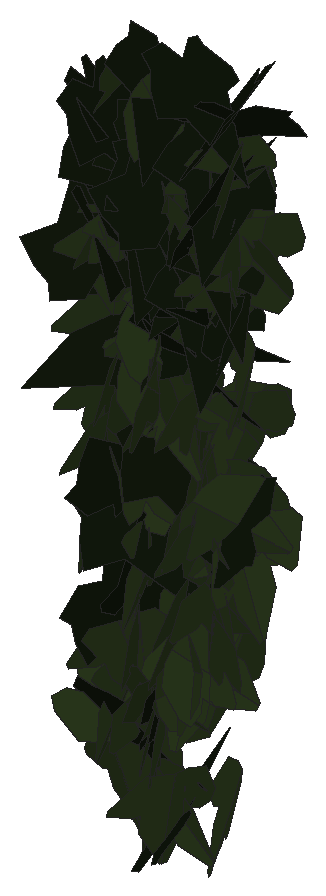
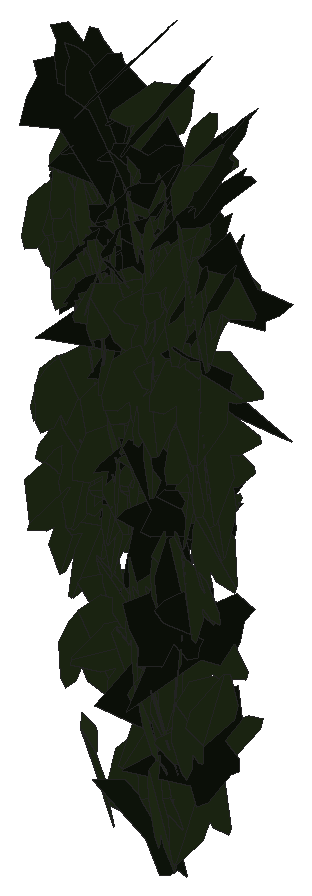
# SketchUp Ruby script. Lengths in inches.
U = 1.inch
M = Sketchup.active_model
def pt(a) = Geom::Point3d.new(a.map { |v| v * U })
def face(e, loops, mat)
  f = e.add_face(loops[0].map { |a| pt(a) })
  loops[1..].each { |l| e.add_face(l.map { |a| pt(a) }).erase! }
  f.material = f.back_material = mat if mat
  f
end
# faces: each face lists its corners as indices into pts; further lists are holes
def faces(e, pts, list, mat = nil) = list.each { |f| face(e, (f[0].is_a?(Array) ? f : [f]).map { |l| l.map { |i| pts[i] } }, mat) }
# xy, xz, yz: faces in a plane at the given z, y or x. An outline is a flat list of corners, or four numbers for a rectangle; further outlines are holes
def ring(l) = l.size == 4 ? [[l[0], l[1]], [l[2], l[1]], [l[2], l[3]], [l[0], l[3]]] : l.each_slice(2).to_a
def flat(e, list, mat, &to3) = list.each { |f| face(e, (f[0].is_a?(Array) ? f : [f]).map { |l| ring(l).map { |u, v| to3.(u, v) } }, mat) }
def xy(e, z, list, mat = nil) = flat(e, list, mat) { |x, y| [x, y, z] }
def xz(e, y, list, mat = nil) = flat(e, list, mat) { |x, z| [x, y, z] }
def yz(e, x, list, mat = nil) = flat(e, list, mat) { |y, z| [x, y, z] }
def lines(e, pts, list) = list.each { |a, b| e.add_line(pt(pts[a]), pt(pts[b])) }
# prism: a flat outline (further loops are holes) pulled along v
def prism(e, loops, v, mat = nil)
  f = face(e, loops, mat); d = Geom::Vector3d.new(v.map { |x| x * U })
  f.pushpull(f.normal.samedirection?(d) ? d.length : -d.length)
end
def box(e, o, s, mat = nil) = prism(e, [[o, [o[0] + s[0], o[1], o[2]], [o[0] + s[0], o[1] + s[1], o[2]], [o[0], o[1] + s[1], o[2]]]], [0, 0, s[2]], mat)
def at(x, y, z, deg = 0) = Geom::Transformation.translation(pt([x, y, z])) * Geom::Transformation.rotation(ORIGIN, Z_AXIS, deg.degrees)
def axes(o, x, y, z) = Geom::Transformation.new([*x, 0, *y, 0, *z, 0, *pt(o).to_a, 1])
def part(name) = M.definitions.add(name)
# library, detail: a bought-in or finely detailed component or shape, given as its bounding box
def library(name, o, s) = part(name).tap { |d| box(d.entities, o, s) }
def detail(e, o, s) = box(e.add_group.entities, o, s)
def put(e, d, t, mat = nil) = e.add_instance(d, t).tap { |i| i.material = mat if mat }
def group(e, t, mat = nil) = e.add_group.tap { |g| g.transformation = t; g.material = mat if mat }.entities
root = M.entities
M.materials.add("efeu1").color = [18, 25, 13]
M.materials.add("efeu2").color = [43, 57, 29]
c1 = part("ivyleaf_10")
p = [[0,0.5,-0.03],[-0.0625,2.02,-0.43],[-0.19,2.01,-0.46],[-0.54,1.05,-0.29],[-0.52,0.625,-0.18],[-0.83,0.76,-0.28],
  [-1.16,0.64,-0.33],[-1.15,0.33,-0.24],[-0.77,-0.39,0.02],[-0.3,-0.51,0.16],[0.04,-0.48,0.23],[-0.02,2.01,-0.4375],
  [-0.06,2.01,-0.43],[0.04,-0.49,0.23],[0.67,-0.49,0.14],[1.38,0.36,-0.2],[1.375,0.51,-0.24],[0.81,0.65,-0.19],
  [0.62,0.59,-0.15],[0.6,1.09,-0.28],[0.5,1.23,-0.31]]
faces(c1.entities,p,[[0,1,2,3,4,5,6,7,8,9,10],[11,12,0,13,14,15,16,17,18,19,20]],"efeu2")
c2 = part("ivyleaf_9")
p = [[1.54,2.16,1.25],[1.36,2.04,1.19],[-0.21,0.99,0.68],[-0.71,1.11,0.82],[-0.85,0.86,0.67],[-0.8,0.17,0.21],
  [-0.9,-0.01,0.1],[-0.67,-0.16,-0.02],[-0.08,-0.08,-0.05],[-0.03,-0.6,-0.4],[0.65,-0.88,-0.66],[0.83,-0.6,-0.49],
  [1.29,-0.42,-0.43],[1.8125,-0.07,-0.26],[1.21,0.44,0.15]]
faces(c2.entities,p,[[0,1,2,3,4,5,6,7,8,9,10,11,12,13,14]],"efeu1")
put(root,c1,axes([25.26,224.34,221.76],[0.24125,-0.40077,-0.17658],[-0.09619,0.14819,-0.46775],[0.42726,0.25966,-0.0056]))
put(root,c2,axes([24.83,224.32,221.36],[-0.37536,-0.25401,0.21115],[0.19137,0.09328,0.45241],[-0.26923,0.42045,0.02719]))
put(root,c1,axes([25.51,224.54,222.11],[0.27688,-0.39865,0.12008],[0.06912,-0.0982,-0.48537],[0.41056,0.28537,0.00073]))
put(root,c1,axes([24.86,224.34,221.39],[-0.44159,0.20009,0.12234],[-0.14457,-0.02688,-0.47789],[-0.18466,-0.45743,0.08159]))
put(root,c1,axes([25.24,224.48,217.3125],[-0.32145,0.27597,-0.26553],[0.17932,-0.19786,-0.42272],[-0.3384,-0.367,0.02824]))
put(root,c2,axes([25.45,224,221.625],[-0.14447,0.35957,-0.31597],[-0.17377,0.26814,0.38458],[0.44602,0.22094,0.04749]))
put(root,c1,axes([25.05,224.46,215.98],[0.49919,-0.02525,-0.01328],[-0.01333,-0.00063,-0.49982],[0.02523,0.49936,-0.0013]))
put(root,c1,axes([24.43,224.48,215.16],[-0.13491,-0.11978,0.46632],[0.48069,-0.00613,0.13749],[-0.02722,0.4854,0.1168]))
put(root,c2,axes([24.39,224.78,220.92],[-0.08197,-0.43899,0.22487],[0.06452,-0.23554,-0.4363],[0.489,-0.04251,0.09526]))
put(root,c1,axes([25.18,224.375,219.25],[0.01017,-0.48387,-0.12558],[0.01167,0.1258,-0.48378],[0.49976,0.00691,0.01386]))
put(root,c1,axes([24.98,224.32,219.89],[-0.30365,0.07084,0.39087],[-0.38961,0.04283,-0.31044],[-0.07746,-0.4931,0.02919]))
put(root,c1,axes([24.76,224.46,214.35],[-0.21336,-0.45182,0.01833],[-0.00763,-0.01666,-0.49966],[0.45213,-0.21349,0.00022]))
put(root,c2,axes([25.3125,224.7,222.08],[-0.10227,-0.48689,0.04975],[0.00111,-0.05106,-0.49738],[0.48943,-0.10162,0.01153]))
put(root,c1,axes([24.6875,224.17,219.3],[0.06707,-0.30622,-0.38953],[-0.03302,0.38945,-0.31184],[0.49438,0.06755,0.03202]))
put(root,c1,axes([25.15,224.25,216],[0.15132,-0.14421,-0.45421],[-0.32558,0.31671,-0.20902],[0.34799,0.35902,0.00195]))
put(root,c2,axes([24.61,224.36,219.71],[0.46299,-0.10613,0.15611],[0.15168,-0.03698,-0.475],[0.11237,0.4872,-0.00205]))
put(root,c1,axes([25.47,224.34,216.55],[-0.39659,0.22791,0.20193],[-0.21896,0.01695,-0.44919],[-0.21159,-0.44472,0.08636]))
put(root,c1,axes([25.48,224.25,217.1],[-0.15098,-0.37738,-0.29119],[0.09597,0.27513,-0.40632],[0.4669,-0.17858,-0.01065]))
put(root,c1,axes([24.64,224.16,220.11],[0.06018,0.36522,0.33615],[0.03586,0.33452,-0.36987],[-0.49507,0.06863,0.01406]))
put(root,c2,axes([24.39,224.77,222.78],[0.00354,-0.46054,0.19466],[-0.00146,-0.19467,-0.46055],[0.49999,0.00269,-0.00272]))
put(root,c1,axes([25.24,224.39,217.71],[-0.0609,-0.47728,-0.13599],[0.0119,0.13557,-0.48112],[0.49614,-0.06183,-0.00515]))
put(root,c2,axes([23.65,224.79,220.55],[0.04918,-0.31313,0.38669],[0.11775,-0.37021,-0.31476],[0.48344,0.12202,0.03733]))
put(root,c2,axes([24.92,224.49,223.15],[0.23115,-0.42908,-0.11163],[0.01092,0.13136,-0.48231],[0.44323,0.22053,0.0701]))
put(root,c2,axes([23.86,224.35,220.375],[-0.48282,-0.05615,0.11718],[0.12087,-0.02853,0.48433],[-0.0477,0.49602,0.04113]))
put(root,c1,axes([24.57,224.53,219.05],[0.32074,-0.04505,0.38092],[0.38124,-0.01716,-0.32304],[0.04218,0.49767,0.02335]))
put(root,c1,axes([24.07,224.48,220.72],[-0.38317,-0.31634,0.05581],[-0.04121,-0.03774,-0.49687],[0.31857,-0.38537,0.00285]))
put(root,c1,axes([23.74,224.69,217.625],[0.11206,-0.4195,0.24792],[0.10255,-0.22839,-0.43281],[0.47637,0.14785,0.03485]))
put(root,c2,axes([24.71,224.24,219.93],[0.39512,0.05725,0.301],[0.28953,0.09099,-0.39736],[-0.10027,0.48831,0.03875]))
put(root,c2,axes([23.8,224.39,222.45],[0.25396,-0.35085,-0.24982],[-0.07832,0.24756,-0.42729],[0.42352,0.25616,0.07079]))
put(root,c1,axes([24.28,224.77,217.05],[0.08985,-0.34157,0.35392],[0.16478,-0.31808,-0.34882],[0.46344,0.17932,0.05541]))
put(root,c1,axes([25.12,224.28,217.94],[0.04081,-0.37013,-0.33367],[0.00971,0.33532,-0.37077],[0.49824,0.02378,0.03456]))
put(root,c1,axes([25.14,224.51,220.23],[-0.36936,-0.07828,0.32778],[-0.31375,-0.09763,-0.37687],[0.12301,-0.48409,0.023]))
put(root,c2,axes([25.12,224.74,220.5],[-0.06218,-0.49558,0.02317],[-0.00601,-0.02259,-0.49945],[0.49608,-0.06239,-0.00314]))
put(root,c2,axes([25.74,224.35,222.94],[-0.23271,0.44253,0.0028],[-0.00126,0.0025,-0.49999],[-0.44254,-0.23272,-0.00005]))
put(root,c1,axes([25.4375,224.3,218.04],[-0.25013,-0.19186,-0.3881],[0.31852,0.22202,-0.31504],[0.29323,-0.40484,0.01116]))
put(root,c2,axes([23.86,224.6,220.97],[0.33738,-0.35707,0.09313],[0.06486,-0.06685,-0.49125],[0.36328,0.34355,0.00121]))
put(root,c2,axes([24.51,224.76,221.38],[-0.10197,-0.48917,0.01782],[0.00351,-0.01893,-0.49963],[0.48948,-0.10177,0.00729]))
put(root,c1,axes([25.7,224.52,219.78],[0.326,-0.36779,-0.09196],[-0.03977,0.08744,-0.49069],[0.37702,0.32724,0.02776]))
put(root,c2,axes([25.28,224.26,220],[-0.44533,0.21409,-0.07647],[-0.07149,0.02776,0.49408],[0.2158,0.45099,0.00589]))
put(root,c1,axes([24.52,224.77,215.28],[0.19891,-0.34066,0.30723],[0.18215,-0.24868,-0.39367],[0.42101,0.26854,0.02517]))
put(root,c1,axes([23.78,224.54,218.36],[0.04873,-0.49514,-0.04964],[-0.01017,0.04888,-0.4975],[0.49752,0.0495,-0.00531]))
put(root,c1,axes([24.71,224.375,219.36],[-0.23916,0.13458,0.41796],[-0.41337,0.09149,-0.26599],[-0.14807,-0.47278,0.0675]))
put(root,c2,axes([25.8,224.43,217.87],[-0.34368,0.25237,0.26114],[-0.21032,0.15479,-0.42639],[-0.29606,-0.40293,-0.00024]))
put(root,c1,axes([24.88,224.67,220.28],[-0.30775,-0.35885,0.16283],[-0.02875,-0.18561,-0.46338],[0.39302,-0.29458,0.09361]))
put(root,c2,axes([24.15,224.29,217.71],[-0.08164,-0.10098,0.48284],[0.41474,0.25091,0.1226],[-0.26707,0.42053,0.04279]))
put(root,c1,axes([24.14,224.46,216],[-0.32735,-0.35016,-0.14222],[0.09847,0.10264,-0.47934],[0.36489,-0.34184,0.00176]))
put(root,c2,axes([24.51,224.66,221.76],[0.00777,-0.47763,-0.14766],[0.02783,0.14787,-0.47682],[0.49916,-0.00081,0.02888]))
put(root,c2,axes([24.22,224.47,217.67],[-0.02552,-0.32017,-0.3832],[0.08958,0.37454,-0.3189],[0.49125,-0.08493,0.03824]))
put(root,c1,axes([24.52,224.63,221.59],[-0.33325,0.28316,-0.24241],[0.13042,-0.21604,-0.43165],[-0.34919,-0.35092,0.07014]))
put(root,c2,axes([24.125,224.6875,219.54],[-0.47321,-0.00043,0.16147],[-0.16146,0.00445,-0.47319],[-0.00103,-0.49998,-0.00435]))
put(root,c2,axes([23.8,224.71,221.78],[0.05314,-0.49257,-0.06743],[-0.00193,0.06761,-0.4954],[0.49716,0.05291,0.00529]))
put(root,c1,axes([25.2,224.24,216.12],[0.06779,0.31975,0.37837],[0.07702,0.37045,-0.32686],[-0.48936,0.1026,0.00097]))
put(root,c1,axes([24.91,224.86,218.25],[-0.12557,0.10903,-0.47154],[0.13904,-0.45849,-0.14304],[-0.46358,-0.16704,0.08482]))
put(root,c1,axes([24.84,224.53,216.71],[0.16659,-0.4593,-0.10627],[-0.01459,0.10763,-0.48806],[0.47121,0.16571,0.02246]))
put(root,c1,axes([24.56,224.33,218.28],[0.09804,0.42707,0.24083],[-0.02348,0.24941,-0.43272],[-0.48973,0.07354,0.06895]))
put(root,c1,axes([24.53,224.43,215.29],[0.03184,-0.445,0.22574],[0.05384,0.22795,0.44175],[-0.49607,-0.00382,0.06244]))
put(root,c2,axes([23.7,224.51,214.93],[0.43907,-0.11117,0.21181],[0.20054,-0.07028,-0.4526],[0.13041,0.48239,-0.01713]))
put(root,c1,axes([23.83,224.875,222.375],[0.02284,0.24019,-0.43793],[-0.06897,-0.43268,-0.2409],[-0.49469,0.07141,0.01337]))
put(root,c1,axes([24.4375,224.67,215.33],[0.27307,-0.41716,0.03753],[0.02365,-0.02937,-0.49858],[0.41818,0.27407,0.00369]))
put(root,c2,axes([24.6,224.58,218.5],[0.09999,-0.42013,-0.25199],[-0.01749,0.25396,-0.43035],[0.48959,0.09487,0.03609]))
put(root,c2,axes([25.25,224.82,221.14],[-0.44032,-0.23676,-0.0081],[0.00736,0.0034,-0.49993],[0.23678,-0.44038,0.00049]))
put(root,c1,axes([24.58,224.38,222.65],[0.07917,0.44159,0.22075],[-0.0195,0.22619,-0.44548],[-0.49331,0.06193,0.05304]))
put(root,c1,axes([23.88,224.86,215.31],[0.0821,-0.39327,0.29765],[0.11869,-0.27713,-0.39889],[0.47872,0.13615,0.04785]))
put(root,c2,axes([24.53,224.73,222.13],[-0.26618,-0.35174,-0.23544],[0.14783,0.18336,-0.44105],[0.39661,-0.3044,0.00638]))
put(root,c2,axes([25.51,224.375,222.65],[-0.17792,0.45133,0.12102],[-0.0544,0.10861,-0.48502],[-0.46409,-0.18576,0.01045]))
put(root,c1,axes([25.47,224.39,220.13],[0.17468,-0.26693,-0.38501],[-0.15766,0.35345,-0.31657],[0.44117,0.232,0.03932]))
put(root,c1,axes([25.38,224.61,222.1],[-0.24956,-0.4306,-0.04799],[0.05643,0.02261,-0.49629],[0.42958,-0.25312,0.03732]))
put(root,c2,axes([25.17,224.75,220.82],[-0.49545,-0.00559,0.06709],[-0.0671,0.0006,-0.49548],[0.00546,-0.49997,-0.00134]))
put(root,c1,axes([24.13,224.8,220.92],[-0.13189,-0.44782,0.17906],[0.02071,-0.19072,-0.46173],[0.48185,-0.11438,0.06885]))
put(root,c1,axes([25.5,224.76,220.58],[-0.07664,-0.47936,0.11975],[-0.00127,-0.12099,-0.48514],[0.49409,-0.07467,0.01733]))
put(root,c1,axes([24.65,224.46,220.02],[0.17674,-0.34712,-0.31348],[-0.08526,0.30559,-0.38645],[0.45988,0.19006,0.04882]))
put(root,c2,axes([25.1,224.81,221.09],[0.09281,-0.49023,-0.03253],[0.01361,0.03566,-0.49854],[0.49112,0.09165,0.01996]))
put(root,c1,axes([23.84,224.58,214.87],[0.22334,0.4461,0.03334],[-0.03207,-0.0212,0.49852],[0.4462,-0.22481,0.01915]))
put(root,c2,axes([23.56,224.59,222.38],[0.38203,-0.30057,-0.11708],[-0.06181,0.1099,-0.48384],[0.31659,0.38416,0.04682]))
put(root,c1,axes([25.47,224.7,221.27],[0.23628,-0.43943,0.03271],[0.11403,0.02513,-0.48618],[0.42564,0.23721,0.11209]))
put(root,c1,axes([23.87,224.59,219.14],[0.21634,-0.42314,-0.15539],[-0.02654,0.16011,-0.47293],[0.44999,0.21288,0.04681]))
put(root,c1,axes([23.94,224.78,217.15],[0.39532,-0.18848,0.24124],[0.23027,-0.07657,-0.43717],[0.20173,0.45674,0.02626]))
put(root,c1,axes([25.41,224.73,220.79],[-0.13542,-0.47892,0.04793],[-0.0009,-0.04954,-0.49754],[0.48131,-0.13484,0.01255]))
put(root,c1,axes([24.375,224.71,214.0625],[0.19611,-0.04222,0.45799],[0.45982,0.00696,-0.19625],[0.0102,0.49817,0.04155]))
put(root,c1,axes([24.98,224.3,215.66],[0.01327,-0.08496,0.49255],[-0.01496,0.49244,0.08534],[-0.4996,-0.017,0.01053]))
put(root,c1,axes([24.57,224.78,216.1],[0.2476,-0.1203,-0.4174],[0.36657,-0.19991,0.27506],[-0.23306,-0.44223,-0.0108]))
put(root,c1,axes([25.38,224.7,221.46],[0.18391,0.43509,-0.16394],[-0.22394,-0.07161,-0.44127],[-0.40746,0.23574,0.16853]))
put(root,c1,axes([24.79,224.5625,216.27],[0.09695,-0.43958,-0.21765],[-0.0314,0.21585,-0.44992],[0.48951,0.1009,0.01424]))
put(root,c1,axes([24.5,224.8,219.375],[-0.37925,-0.26355,0.1916],[-0.09462,-0.19227,-0.45175],[0.3118,-0.37891,0.09596]))
put(root,c1,axes([25.3125,224.77,214.4],[0.35035,-0.35469,0.03813],[0.02032,-0.03351,-0.49846],[0.35615,0.35082,-0.00907]))
put(root,c1,axes([24.21,224.53,216.14],[0.21001,-0.38059,-0.24708],[-0.01428,0.26658,-0.42277],[0.45353,0.18463,0.1011]))
put(root,c1,axes([24.53,224.61,218.94],[0.02757,-0.47627,-0.1497],[0.00834,0.15035,-0.47679],[0.49917,0.0238,0.01623]))
put(root,c1,axes([23.78,224.74,218.85],[-0.16139,-0.47259,0.02464],[-0.00936,-0.02284,-0.49939],[0.47314,-0.16166,-0.00147]))
put(root,c1,axes([24.64,224.84,221.57],[0.21437,-0.43143,0.13385],[0.11135,-0.09312,-0.47847],[0.43777,0.23495,0.05616]))
put(root,c1,axes([24.28,224.53,217.91],[0.04211,0.02242,0.49772],[0.40365,0.29126,-0.04728],[-0.29205,0.40579,0.00643]))
put(root,c1,axes([24.39,224.47,215.31],[-0.16046,-0.31249,-0.35582],[0.15025,0.32268,-0.35114],[0.44909,-0.21961,-0.00965]))
put(root,c1,axes([25.46,224.77,221.67],[-0.09269,-0.49102,0.01752],[-0.00492,-0.0169,-0.49969],[0.49131,-0.0928,-0.0017]))
put(root,c1,axes([23.9,224.66,214.39],[-0.49018,0.08387,-0.05187],[0.05063,-0.01166,-0.49729],[-0.08462,-0.49278,0.00294]))
put(root,c1,axes([24.35,224.79,221.18],[0.10684,-0.48836,0.00956],[0.00518,-0.00865,-0.4999],[0.48842,0.10692,0.00321]))
put(root,c1,axes([25.24,224.76,220.7],[-0.27132,0.37806,-0.1829],[0.09677,-0.15561,-0.46521],[-0.40868,-0.28784,0.01127]))
put(root,c1,axes([25.57,224.62,217.4],[0.05865,0.49208,0.06646],[0.01291,0.06538,-0.49554],[-0.49638,0.05984,-0.00503]))
put(root,c1,axes([23.78,224.71,220.83],[0.06489,-0.48714,-0.09209],[0.00004,0.09288,-0.4913],[0.49577,0.06376,0.0121]))
put(root,c1,axes([25.67,224.85,217.79],[0.22752,0.28377,-0.34309],[-0.33353,-0.14661,-0.34243],[-0.29494,0.38468,0.12258]))
put(root,c1,axes([24.43,224.62,220.92],[0.14411,-0.43412,-0.20192],[0.05562,0.22462,-0.44323],[0.47554,0.10528,0.11303]))
put(root,c2,axes([23.89,224.45,216.52],[0.04994,-0.12353,-0.48192],[-0.12937,0.46445,-0.13246],[0.48038,0.13792,0.01443]))
put(root,c2,axes([25.52,224.57,222.73],[0.16226,0.40901,-0.23746],[-0.22939,-0.15148,-0.41765],[-0.41359,0.24448,0.13848]))
put(root,c1,axes([25.45,224.79,221.39],[-0.0467,-0.49781,0.00089],[0.00029,-0.00092,-0.5],[0.49781,-0.0467,0.00038]))
put(root,c1,axes([24.87,224.77,218.35],[-0.45273,-0.20482,0.0555],[-0.02401,-0.0805,-0.49289],[0.21085,-0.44896,0.06306]))
put(root,c1,axes([25.89,224.72,220.74],[-0.27818,0.11696,-0.39866],[-0.39129,0.08752,0.29872],[0.13966,0.47818,0.04284]))
put(root,c1,axes([25.52,224.92,219.08],[-0.1892,-0.42158,0.19098],[-0.0148,-0.2007,-0.45771],[0.46259,-0.17885,0.06347]))
put(root,c1,axes([23.84,224.72,220.79],[-0.41702,-0.26085,-0.08976],[0.09257,0.02093,-0.49091],[0.25986,-0.42605,0.03084]))
put(root,c1,axes([25.52,224.81,219.07],[-0.27398,-0.41218,0.07103],[-0.04426,-0.05586,-0.49489],[0.4159,-0.27747,-0.00588]))
put(root,c1,axes([24.86,224.59,215.71],[-0.18341,0.21636,0.41176],[-0.41822,0.11704,-0.24778],[-0.20361,-0.43531,0.13804]))
put(root,c1,axes([25.68,224.83,221.22],[-0.21757,-0.44615,0.06015],[-0.00523,-0.0643,-0.49582],[0.45015,-0.21638,0.02331]))
put(root,c1,axes([25.22,224.96,216],[-0.09781,-0.44774,0.1999],[0.04876,-0.21171,-0.45033],[0.48791,-0.0686,0.08508]))
put(root,c2,axes([24.61,224.36,215.23],[0.07208,0.13729,0.47535],[0.15995,0.44811,-0.15367],[-0.46821,0.17422,0.02068]))
put(root,c1,axes([24.36,224.44,219.25],[-0.01064,0.32854,0.37676],[0.0002,0.37685,-0.32861],[-0.49989,-0.00684,-0.00815]))
put(root,c1,axes([25.31,224.82,221.43],[0.12105,-0.48458,-0.02302],[0.00351,0.0246,-0.49938],[0.48511,0.12074,0.00936]))
put(root,c1,axes([24,224.48,218.37],[-0.17185,0.25251,0.39586],[-0.25979,0.3,-0.30415],[-0.39112,-0.31022,0.02809]))
put(root,c1,axes([25.0625,224.79,221.49],[0.33473,-0.36942,-0.03855],[0.03938,0.08689,-0.49081],[0.36934,0.32554,0.08726]))
put(root,c1,axes([23.95,224.82,221.42],[0.21173,-0.45069,-0.0453],[0.00444,0.05207,-0.49726],[0.45294,0.21017,0.02606]))
put(root,c2,axes([24.55,224.49,213.57],[-0.24064,0.43487,-0.05459],[-0.02973,0.04594,0.497],[0.43728,0.24244,0.00375]))
put(root,c1,axes([23.77,224.78,219.66],[-0.34319,-0.36328,-0.01575],[0.01044,0.0118,-0.49975],[0.36348,-0.34334,-0.00052]))
put(root,c1,axes([24.77,224.83,220.31],[0.43305,0.22296,-0.11295],[-0.11869,-0.01539,-0.48546],[-0.21996,0.44727,0.0396]))
put(root,c1,axes([23.97,224.74,221.13],[-0.01509,0.49977,0.0018],[-0.02763,0.00097,-0.49923],[-0.49901,-0.01516,0.02759]))
put(root,c1,axes([24.26,224.91,214.27],[0.19811,-0.4551,0.06029],[0.0449,-0.04614,-0.49584],[0.45688,0.20187,0.02258]))
put(root,c2,axes([24.01,224.95,216.32],[0.17446,0.2916,0.36678],[-0.19126,-0.31298,0.3398],[0.42776,-0.25887,0.00234]))
put(root,c1,axes([25.37,224.76,218.23],[-0.49852,-0.03341,-0.01905],[0.01899,0.00147,-0.49964],[0.03345,-0.49888,-0.0002]))
put(root,c1,axes([24.45,224.85,219.55],[-0.29207,-0.40418,0.0365],[-0.02091,-0.02993,-0.49867],[0.40528,-0.29282,0.00058]))
put(root,c1,axes([24.2,224.85,220.24],[-0.45544,0.0043,-0.20628],[0.1996,-0.11742,-0.44314],[-0.05226,-0.486,0.10524]))
put(root,c1,axes([23.83,224.91,217.21],[0.44253,-0.19949,0.11989],[0.12275,-0.01877,-0.48433],[0.19774,0.4581,0.03236]))
